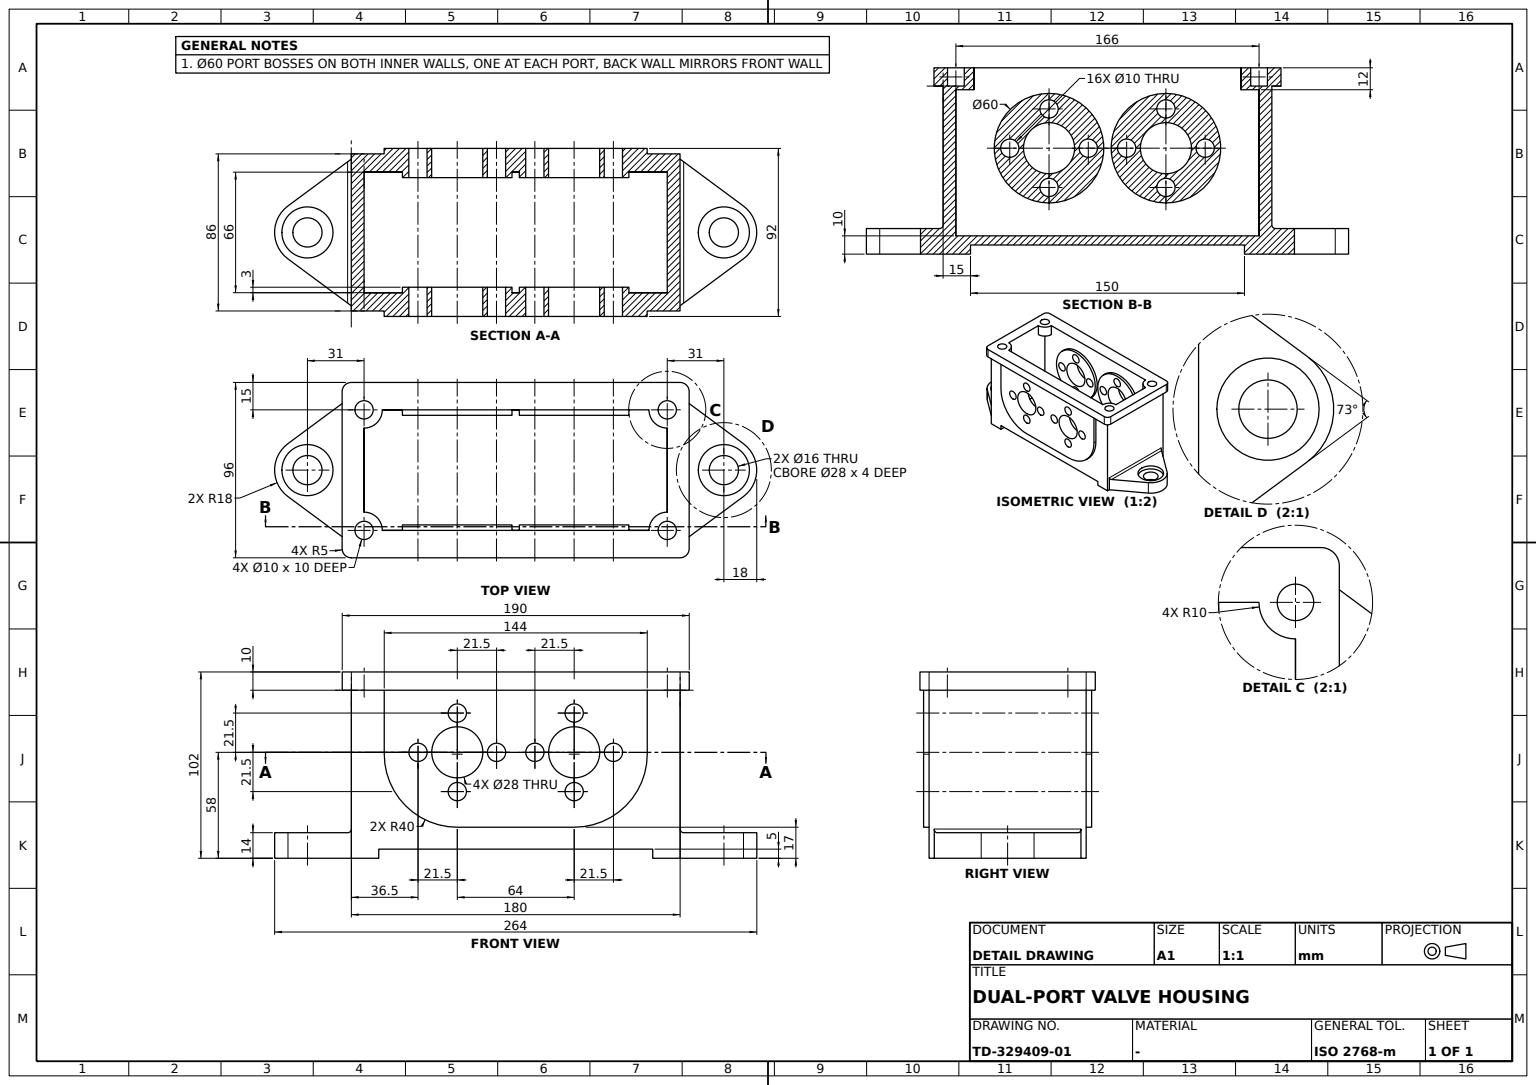
solid
v1 (-88,-33,92)
e1 v1 v1 CIRCLE(AX(P(-83,-33,92),D(0,0,-1),D(-1,0,0)),5) rev
face PLANE(AX(P(-83,-33,92),D(0,0,-1),D(-1,0,0))) rev [e1]
v2 (-90,-48,92)
v3 (-95,-43,92)
e2 v2 v3 CIRCLE(AX(P(-90,-43,92),D(0,0,1),D(1,0,0)),5) rev
v4 (-90,-48,102)
e3 v4 v2 LINE
v5 (-95,-43,102)
e4 v5 v4 CIRCLE(AX(P(-90,-43,102),D(0,0,1),D(1,0,0)),5)
e5 v3 v5 LINE
face CYL(AX(P(-90,-43,102),D(0,0,-1),D(-1,0,0)),5) [-e2 -e3 -e4 -e5]
v6 (-83,33,90)
v7 (-73,33,90)
e6 v6 v7 LINE
v8 (-83,23,90)
e7 v7 v8 CIRCLE(AX(P(-83,33,90),D(0,0,-1),D(1,0,0)),10)
e8 v8 v6 LINE
face PLANE(AX(P(-83,33,90),D(0,0,-1),D(-1,0,0))) [e6 e7 e8]
v9 (32,30,74.5)
e9 v9 v9 CIRCLE(AX(P(32,30,79.5),D(0,-1,0),D(0,0,-1)),5)
v10 (32,46,74.5)
e10 v10 v10 CIRCLE(AX(P(32,46,79.5),D(0,-1,0),D(0,0,-1)),5)
face CYL(AX(P(32,46,79.5),D(0,-1,0),D(0,0,-1)),5) rev [e9] [-e10]
v11 (100,0,14)
e11 v11 v11 CIRCLE(AX(P(114,0,14),D(0,0,-1),D(-1,0,0)),14)
v12 (100,0,10)
e12 v12 v12 CIRCLE(AX(P(114,0,10),D(0,0,-1),D(-1,0,0)),14) rev
face CYL(AX(P(114,0,14),D(0,0,-1),D(-1,0,0)),14) rev [-e11] [-e12]
v13 (53.5,30,53)
e13 v13 v13 CIRCLE(AX(P(53.5,30,58),D(0,-1,0),D(0,0,-1)),5)
v14 (53.5,46,53)
e14 v14 v14 CIRCLE(AX(P(53.5,46,58),D(0,-1,0),D(0,0,-1)),5)
face CYL(AX(P(53.5,46,58),D(0,-1,0),D(0,0,-1)),5) rev [e13] [-e14]
v15 (-95,43,102)
e15 v15 v5 LINE
v16 (-95,43,92)
e16 v15 v16 LINE
e17 v16 v3 LINE
face PLANE(AX(P(-95,48,102),D(1,0,0),D(0,0,-1))) rev [-e15 e16 e17 e5]
v17 (-32,30,31.5)
e18 v17 v17 CIRCLE(AX(P(-32,30,36.5),D(0,-1,0),D(0,0,-1)),5)
v18 (-32,30,74.5)
e19 v18 v18 CIRCLE(AX(P(-32,30,79.5),D(0,-1,0),D(0,0,-1)),5)
v19 (-10.5,30,53)
e20 v19 v19 CIRCLE(AX(P(-10.5,30,58),D(0,-1,0),D(0,0,-1)),5)
v20 (-32,30,72)
e21 v20 v20 CIRCLE(AX(P(-32,30,58),D(0,1,0),D(0,0,1)),14)
v21 (-53.5,30,53)
e22 v21 v21 CIRCLE(AX(P(-53.5,30,58),D(0,-1,0),D(0,0,-1)),5)
v22 (-2,30,58)
e23 v22 v22 CIRCLE(AX(P(-32,30,58),D(0,-1,0),D(1,0,0)),30)
face PLANE(AX(P(-32,30,58),D(0,-1,0),D(0,0,-1))) [-e18] [-e19] [-e20] [e21] [-e22] [e23]
v23 (73,33,90)
v24 (83,23,90)
e24 v23 v24 CIRCLE(AX(P(83,33,90),D(0,0,1),D(-1,0,0)),10)
v25 (83,23,102)
e25 v24 v25 LINE
v26 (73,33,102)
e26 v26 v25 CIRCLE(AX(P(83,33,102),D(0,0,1),D(-1,0,0)),10)
e27 v23 v26 LINE
face CYL(AX(P(83,33,90),D(0,0,1),D(1,0,0)),10) [e24 e25 -e26 -e27]
v27 (-122,0,10)
e28 v27 v27 CIRCLE(AX(P(-114,0,10),D(0,0,-1),D(-1,0,0)),8) rev
v28 (-128,0,10)
e29 v28 v28 CIRCLE(AX(P(-114,0,10),D(0,0,-1),D(-1,0,0)),14) rev
face PLANE(AX(P(-114,0,10),D(0,0,-1),D(-1,0,0))) rev [-e28] [e29]
v29 (78,-33,92)
e30 v29 v29 CIRCLE(AX(P(83,-33,92),D(0,0,-1),D(-1,0,0)),5) rev
face PLANE(AX(P(83,-33,92),D(0,0,-1),D(-1,0,0))) rev [e30]
v30 (-10.5,46,53)
e31 v30 v30 CIRCLE(AX(P(-10.5,46,58),D(0,-1,0),D(0,0,-1)),5)
face CYL(AX(P(-10.5,46,58),D(0,-1,0),D(0,0,-1)),5) rev [-e31] [e20]
v31 (-88,-33,102)
e32 v31 v31 CIRCLE(AX(P(-83,-33,102),D(0,0,-1),D(-1,0,0)),5)
face CYL(AX(P(-83,-33,102),D(0,0,-1),D(-1,0,0)),5) rev [-e32] [-e1]
v32 (90,-40.151112,0)
v33 (124.70681,-14.469423,0)
e33 v32 v33 LINE
v34 (124.70681,-14.469423,14)
e34 v34 v33 LINE
v35 (92,-38.67119,14)
e35 v35 v34 LINE
v36 (90,-40.151112,16)
e36 v35 v36 ELLIPSE(AX(P(92,-38.67119,16),D(-0.594822787,0.803856861,0),D(0.803856861,0.594822787,0)),2.488005,2)
e37 v36 v32 LINE
face PLANE(AX(P(90,-40.151112,14),D(-0.594822787,0.803856861,0),D(-0.803856861,-0.594822787,0))) rev [e33 -e34 -e35 e36 e37]
v37 (-73,-33,90)
v38 (-83,-23,90)
e38 v37 v38 CIRCLE(AX(P(-83,-33,90),D(0,0,1),D(1,0,0)),10)
v39 (-83,-33,90)
e39 v39 v37 LINE
e40 v38 v39 LINE
face PLANE(AX(P(-83,-33,90),D(0,0,1),D(1,0,0))) rev [-e38 -e39 -e40]
v40 (-90,48,92)
v41 (-90,48,102)
e41 v40 v41 LINE
v42 (90,48,102)
e42 v42 v41 LINE
v43 (90,48,92)
e43 v42 v43 LINE
e44 v43 v40 LINE
face PLANE(AX(P(95,48,102),D(0,-1,0),D(0,0,-1))) rev [e41 -e42 e43 e44]
v44 (83,33,90)
e45 v44 v23 LINE
e46 v24 v44 LINE
face PLANE(AX(P(83,33,90),D(0,0,1),D(1,0,0))) rev [-e24 -e45 -e46]
v45 (-124.70681,-14.469423,14)
v46 (-124.70681,14.469423,14)
e47 v45 v46 CIRCLE(AX(P(-114,0,14),D(0,0,-1),D(-1,0,0)),18)
v47 (-92,-38.67119,14)
e48 v47 v45 LINE
v48 (-92,38.67119,14)
e49 v47 v48 LINE
e50 v46 v48 LINE
v49 (-128,0,14)
e51 v49 v49 CIRCLE(AX(P(-114,0,14),D(0,0,-1),D(-1,0,0)),14)
face PLANE(AX(P(-114,0,14),D(0,0,-1),D(-1,0,0))) rev [-e47 -e48 e49 -e50] [e51]
v50 (-32,-46,17)
v51 (-32,-43,17)
e52 v50 v51 LINE
v52 (-72,-46,57)
e53 v52 v50 CIRCLE(AX(P(-32,-46,57),D(0,-1,0),D(1,0,0)),40)
v53 (-72,-43,57)
e54 v52 v53 LINE
e55 v51 v53 CIRCLE(AX(P(-32,-43,57),D(0,-1,0),D(0,0,-1)),40) rev
face CYL(AX(P(-32,-46,57),D(0,1,0),D(0,0,1)),40) [-e52 -e53 e54 -e55]
v54 (90,-48,102)
v55 (95,-43,102)
e56 v54 v55 CIRCLE(AX(P(90,-43,102),D(0,0,1),D(1,0,0)),5)
v56 (90,-48,92)
e57 v56 v54 LINE
v57 (95,-43,92)
e58 v57 v56 CIRCLE(AX(P(90,-43,92),D(0,0,1),D(1,0,0)),5) rev
e59 v55 v57 LINE
face CYL(AX(P(90,-43,102),D(0,0,-1),D(-1,0,0)),5) [-e56 -e57 -e58 -e59]
v58 (124.70681,14.469423,0)
v59 (90,40.151112,0)
e60 v58 v59 LINE
v60 (90,40.151112,16)
e61 v60 v59 LINE
v61 (92,38.67119,14)
e62 v60 v61 ELLIPSE(AX(P(92,38.67119,16),D(-0.594822787,-0.803856861,0),D(-0.803856861,0.594822787,0)),2.488005,2)
v62 (124.70681,14.469423,14)
e63 v62 v61 LINE
e64 v62 v58 LINE
face PLANE(AX(P(124.70681,14.469423,14),D(-0.594822787,-0.803856861,0),D(0.803856861,-0.594822787,0))) rev [e60 -e61 e62 -e63 e64]
v63 (-73,-33,102)
e65 v37 v63 LINE
v64 (-83,-23,102)
e66 v38 v64 LINE
e67 v63 v64 CIRCLE(AX(P(-83,-33,102),D(0,0,1),D(1,0,0)),10)
face CYL(AX(P(-83,-33,90),D(0,0,1),D(1,0,0)),10) [-e65 e38 e66 -e67]
v65 (-32,-30,74.5)
e68 v65 v65 CIRCLE(AX(P(-32,-30,79.5),D(0,-1,0),D(0,0,-1)),5)
v66 (-32,-46,74.5)
e69 v66 v66 CIRCLE(AX(P(-32,-46,79.5),D(0,-1,0),D(0,0,-1)),5)
face CYL(AX(P(-32,46,79.5),D(0,-1,0),D(0,0,-1)),5) rev [-e68] [e69]
v67 (-32,-33,28)
e70 v67 v67 CIRCLE(AX(P(-32,-33,58),D(0,-1,0),D(0,0,-1)),30)
v68 (32,-33,28)
e71 v68 v68 CIRCLE(AX(P(32,-33,58),D(0,-1,0),D(0,0,-1)),30)
v69 (83,-33,10)
v70 (83,-33,90)
e72 v69 v70 LINE
v71 (-83,-33,10)
e73 v71 v69 LINE
e74 v71 v39 LINE
v72 (73,-33,102)
e75 v63 v72 LINE
v73 (73,-33,90)
e76 v73 v72 LINE
e77 v70 v73 LINE
face PLANE(AX(P(83,-33,123),D(0,-1,0),D(0,0,-1))) rev [e70] [e71] [-e72 -e73 e74 e39 e65 e75 -e76 -e77]
v74 (32,-30,74.5)
e78 v74 v74 CIRCLE(AX(P(32,-30,79.5),D(0,-1,0),D(0,0,-1)),5)
v75 (32,-46,74.5)
e79 v75 v75 CIRCLE(AX(P(32,-46,79.5),D(0,-1,0),D(0,0,-1)),5)
face CYL(AX(P(32,46,79.5),D(0,-1,0),D(0,0,-1)),5) rev [-e78] [e79]
v76 (62,-30,58)
e80 v76 v76 CIRCLE(AX(P(32,-30,58),D(0,-1,0),D(1,0,0)),30)
face CYL(AX(P(32,-30,58),D(0,-1,0),D(0,0,-1)),30) [e80] [-e71]
v77 (-88,33,92)
e81 v77 v77 CIRCLE(AX(P(-83,33,92),D(0,0,-1),D(-1,0,0)),5) rev
face PLANE(AX(P(-83,33,92),D(0,0,-1),D(-1,0,0))) rev [e81]
v78 (-72,-46,92)
e82 v78 v52 LINE
v79 (-72,-43,92)
e83 v78 v79 LINE
e84 v53 v79 LINE
face PLANE(AX(P(-72,-46,92),D(1,0,0),D(0,0,-1))) rev [-e82 e83 -e84 -e54]
v80 (95,43,92)
e85 v57 v80 LINE
v81 (95,43,102)
e86 v80 v81 LINE
e87 v55 v81 LINE
face PLANE(AX(P(95,-48,102),D(-1,0,0),D(0,0,1))) rev [e85 e86 -e87 e59]
v82 (106,0,10)
e88 v82 v82 CIRCLE(AX(P(114,0,10),D(0,0,-1),D(-1,0,0)),8) rev
face PLANE(AX(P(114,0,10),D(0,0,-1),D(-1,0,0))) rev [-e88] [e12]
v83 (106,0,0)
e89 v83 v83 CIRCLE(AX(P(114,0,0),D(0,0,-1),D(-1,0,0)),8)
face CYL(AX(P(114,0,-67.414906),D(0,0,-1),D(-1,0,0)),8) rev [e89] [e88]
v84 (-2,-30,58)
e90 v84 v84 CIRCLE(AX(P(-32,-30,58),D(0,-1,0),D(1,0,0)),30)
v85 (-10.5,-30,53)
e91 v85 v85 CIRCLE(AX(P(-10.5,-30,58),D(0,-1,0),D(0,0,-1)),5)
v86 (-53.5,-30,53)
e92 v86 v86 CIRCLE(AX(P(-53.5,-30,58),D(0,-1,0),D(0,0,-1)),5)
v87 (-32,-30,44)
e93 v87 v87 CIRCLE(AX(P(-32,-30,58),D(0,-1,0),D(0,0,-1)),14)
v88 (-32,-30,31.5)
e94 v88 v88 CIRCLE(AX(P(-32,-30,36.5),D(0,-1,0),D(0,0,-1)),5)
face PLANE(AX(P(-32,-30,58),D(0,-1,0),D(0,0,-1))) rev [-e90] [e91] [e92] [e93] [e68] [e94]
v89 (-90,40.151112,0)
v90 (-90,43,0)
e95 v89 v90 LINE
v91 (-75,43,0)
e96 v90 v91 LINE
v92 (-75,-43,0)
e97 v92 v91 LINE
v93 (-90,-43,0)
e98 v92 v93 LINE
v94 (-90,-40.151112,0)
e99 v93 v94 LINE
v95 (-124.70681,-14.469423,0)
e100 v94 v95 LINE
v96 (-124.70681,14.469423,0)
e101 v95 v96 CIRCLE(AX(P(-114,0,0),D(0,0,-1),D(-1,0,0)),18)
e102 v96 v89 LINE
v97 (-122,0,0)
e103 v97 v97 CIRCLE(AX(P(-114,0,0),D(0,0,-1),D(-1,0,0)),8)
face PLANE(AX(P(0,0,0),D(0,0,-1),D(-1,0,0))) [e95 e96 -e97 e98 e99 e100 e101 e102] [-e103]
e104 v33 v58 CIRCLE(AX(P(114,0,0),D(0,0,1),D(1,0,0)),18)
v98 (90,-43,0)
e105 v32 v98 LINE
v99 (75,-43,0)
e106 v98 v99 LINE
v100 (75,43,0)
e107 v100 v99 LINE
v101 (90,43,0)
e108 v100 v101 LINE
e109 v101 v59 LINE
face PLANE(AX(P(0,0,0),D(0,0,-1),D(-1,0,0))) [-e89] [-e104 -e33 e105 e106 -e107 e108 e109 -e60]
v102 (32,46,44)
e110 v102 v102 CIRCLE(AX(P(32,46,58),D(0,-1,0),D(0,0,-1)),14)
v103 (32,30,72)
e111 v103 v103 CIRCLE(AX(P(32,30,58),D(0,1,0),D(0,0,1)),14)
face CYL(AX(P(32,30,58),D(0,1,0),D(0,0,1)),14) rev [-e110] [-e111]
e112 v2 v56 LINE
e113 v4 v54 LINE
face PLANE(AX(P(-95,-48,102),D(0,1,0),D(0,0,1))) rev [e112 e57 -e113 e3]
v104 (-32,46,74.5)
e114 v104 v104 CIRCLE(AX(P(-32,46,79.5),D(0,-1,0),D(0,0,-1)),5)
face CYL(AX(P(-32,46,79.5),D(0,-1,0),D(0,0,-1)),5) rev [e19] [-e114]
v105 (83,-23,90)
e115 v73 v105 CIRCLE(AX(P(83,-33,90),D(0,0,-1),D(-1,0,0)),10)
e116 v105 v70 LINE
face PLANE(AX(P(83,-33,90),D(0,0,-1),D(-1,0,0))) [e77 e115 e116]
face CYL(AX(P(-114,0,-67.414906),D(0,0,-1),D(-1,0,0)),8) rev [e28] [e103]
v106 (-32,-46,31.5)
e117 v106 v106 CIRCLE(AX(P(-32,-46,36.5),D(0,-1,0),D(0,0,-1)),5)
face CYL(AX(P(-32,46,36.5),D(0,-1,0),D(0,0,-1)),5) rev [-e94] [e117]
v107 (-72,46,57)
v108 (-32,46,17)
e118 v107 v108 CIRCLE(AX(P(-32,46,57),D(0,-1,0),D(1,0,0)),40)
v109 (-32,43,17)
e119 v109 v108 LINE
v110 (-72,43,57)
e120 v110 v109 CIRCLE(AX(P(-32,43,57),D(0,1,0),D(0,0,1)),40) rev
e121 v110 v107 LINE
face CYL(AX(P(-32,-46,57),D(0,1,0),D(0,0,1)),40) [e118 -e119 -e120 e121]
v111 (-88,33,102)
e122 v111 v111 CIRCLE(AX(P(-83,33,102),D(0,0,-1),D(-1,0,0)),5)
v112 (-73,33,102)
e123 v26 v112 LINE
v113 (83,-23,102)
e124 v113 v25 LINE
e125 v72 v113 CIRCLE(AX(P(83,-33,102),D(0,0,-1),D(-1,0,0)),10)
v114 (-83,23,102)
e126 v114 v64 LINE
e127 v112 v114 CIRCLE(AX(P(-83,33,102),D(0,0,-1),D(1,0,0)),10)
v115 (78,-33,102)
e128 v115 v115 CIRCLE(AX(P(83,-33,102),D(0,0,-1),D(-1,0,0)),5)
v116 (78,33,102)
e129 v116 v116 CIRCLE(AX(P(83,33,102),D(0,0,-1),D(-1,0,0)),5)
e130 v81 v42 CIRCLE(AX(P(90,43,102),D(0,0,1),D(1,0,0)),5)
e131 v41 v15 CIRCLE(AX(P(-90,43,102),D(0,0,1),D(1,0,0)),5)
face PLANE(AX(P(0,0,102),D(0,0,1),D(1,0,0))) [e32] [e122] [-e123 e26 -e124 -e125 -e75 e67 -e126 -e127] [e128] [e129] [e130 e42 e131 e15 e4 e113 e56 e87]
e132 v16 v40 CIRCLE(AX(P(-90,43,92),D(0,0,1),D(1,0,0)),5) rev
e133 v43 v80 CIRCLE(AX(P(90,43,92),D(0,0,1),D(1,0,0)),5) rev
v117 (-90,43,92)
v118 (-72,43,92)
e134 v117 v118 LINE
v119 (-90,-43,92)
e135 v119 v117 LINE
e136 v79 v119 LINE
v120 (72,-46,92)
e137 v120 v78 LINE
v121 (72,-43,92)
e138 v120 v121 LINE
v122 (90,-43,92)
e139 v122 v121 LINE
v123 (90,43,92)
e140 v123 v122 LINE
v124 (72,43,92)
e141 v124 v123 LINE
v125 (72,46,92)
e142 v124 v125 LINE
v126 (-72,46,92)
e143 v125 v126 LINE
e144 v118 v126 LINE
face PLANE(AX(P(0,0,92),D(0,0,1),D(1,0,0))) rev [-e112 e2 -e17 e132 -e44 e133 -e85 e58] [-e134 -e135 -e136 -e83 -e137 e138 -e139 -e140 -e141 e142 e143 -e144]
e145 v123 v101 LINE
v127 (75,43,5)
e146 v127 v100 LINE
v128 (-75,43,5)
e147 v128 v127 LINE
e148 v91 v128 LINE
e149 v117 v90 LINE
e150 v118 v110 LINE
v129 (32,43,17)
e151 v109 v129 LINE
v130 (72,43,57)
e152 v129 v130 CIRCLE(AX(P(32,43,57),D(0,1,0),D(0,0,1)),40) rev
e153 v130 v124 LINE
face PLANE(AX(P(-90,43,92),D(0,1,0),D(0,0,1))) [e145 -e108 -e146 -e147 -e148 -e96 -e149 e134 e150 e120 e151 e152 e153 e141]
v131 (32,46,17)
e154 v129 v131 LINE
v132 (72,46,57)
e155 v131 v132 CIRCLE(AX(P(32,46,57),D(0,-1,0),D(1,0,0)),40)
e156 v130 v132 LINE
face CYL(AX(P(32,-46,57),D(0,1,0),D(0,0,1)),40) [e154 e155 -e156 -e152]
e157 v34 v62 CIRCLE(AX(P(114,0,14),D(0,0,1),D(1,0,0)),18)
e158 v61 v35 LINE
face PLANE(AX(P(114,0,14),D(0,0,1),D(1,0,0))) [e11] [e157 e63 e158 e35]
v133 (10.5,46,53)
e159 v133 v133 CIRCLE(AX(P(10.5,46,58),D(0,-1,0),D(0,0,-1)),5)
v134 (10.5,30,53)
e160 v134 v134 CIRCLE(AX(P(10.5,30,58),D(0,-1,0),D(0,0,-1)),5)
face CYL(AX(P(10.5,46,58),D(0,-1,0),D(0,0,-1)),5) rev [-e159] [e160]
face CYL(AX(P(-32,-30,58),D(0,-1,0),D(0,0,-1)),30) [e90] [-e70]
v135 (78,33,92)
e161 v135 v135 CIRCLE(AX(P(83,33,92),D(0,0,-1),D(-1,0,0)),5) rev
face CYL(AX(P(83,33,102),D(0,0,-1),D(-1,0,0)),5) rev [-e129] [-e161]
e162 v8 v114 LINE
e163 v7 v112 LINE
face CYL(AX(P(-83,33,90),D(0,0,1),D(1,0,0)),10) [e127 -e162 -e7 e163]
v136 (-75,-43,5)
e164 v128 v136 LINE
v137 (75,-43,5)
e165 v127 v137 LINE
e166 v137 v136 LINE
face PLANE(AX(P(-75,-50,5),D(0,0,1),D(1,0,0))) rev [-e164 e147 e165 e166]
v138 (72,-46,57)
e167 v138 v120 LINE
v139 (72,-43,57)
e168 v138 v139 LINE
e169 v121 v139 LINE
face PLANE(AX(P(72,-46,57),D(-1,0,0),D(0,0,1))) rev [-e138 -e167 e168 -e169]
v140 (32,-46,17)
e170 v50 v140 LINE
v141 (32,-43,17)
e171 v141 v51 LINE
e172 v140 v141 LINE
face PLANE(AX(P(-32,-46,17),D(0,0,1),D(1,0,0))) rev [-e170 e52 -e171 -e172]
e173 v126 v107 LINE
face PLANE(AX(P(-72,-46,92),D(1,0,0),D(0,0,-1))) rev [e173 -e121 -e150 e144]
e174 v108 v131 LINE
face PLANE(AX(P(-32,-46,17),D(0,0,1),D(1,0,0))) rev [-e154 -e151 e119 e174]
v142 (-53.5,46,53)
e175 v142 v142 CIRCLE(AX(P(-53.5,46,58),D(0,-1,0),D(0,0,-1)),5)
v143 (-32,46,44)
e176 v143 v143 CIRCLE(AX(P(-32,46,58),D(0,-1,0),D(0,0,-1)),14)
v144 (-32,46,31.5)
e177 v144 v144 CIRCLE(AX(P(-32,46,36.5),D(0,-1,0),D(0,0,-1)),5)
v145 (32,46,31.5)
e178 v145 v145 CIRCLE(AX(P(32,46,36.5),D(0,-1,0),D(0,0,-1)),5)
e179 v132 v125 LINE
face PLANE(AX(P(-32,46,57),D(0,-1,0),D(0,0,-1))) rev [e10] [e31] [e175] [e176] [e177] [e14] [e159] [e110] [e178] [-e174 -e118 -e173 -e143 -e179 -e155] [e114]
face CYL(AX(P(-53.5,46,58),D(0,-1,0),D(0,0,-1)),5) rev [e22] [-e175]
e180 v36 v60 LINE
e181 v122 v98 LINE
face PLANE(AX(P(90,43,92),D(1,0,0),D(0,0,-1))) [-e37 e180 e61 -e109 -e145 e140 e181 -e105]
v146 (-32,33,88)
e182 v146 v146 CIRCLE(AX(P(-32,33,58),D(0,1,0),D(0,0,1)),30)
face CYL(AX(P(-32,43,58),D(0,-1,0),D(0,0,-1)),30) [-e23] [-e182]
v147 (10.5,-46,53)
e183 v147 v147 CIRCLE(AX(P(10.5,-46,58),D(0,-1,0),D(0,0,-1)),5)
v148 (10.5,-30,53)
e184 v148 v148 CIRCLE(AX(P(10.5,-30,58),D(0,-1,0),D(0,0,-1)),5)
face CYL(AX(P(10.5,46,58),D(0,-1,0),D(0,0,-1)),5) rev [e183] [-e184]
face CYL(AX(P(-32,30,58),D(0,1,0),D(0,0,1)),14) rev [-e176] [-e21]
face CYL(AX(P(-90,43,102),D(0,0,-1),D(-1,0,0)),5) [-e131 -e41 -e132 -e16]
face CYL(AX(P(83,-33,102),D(0,0,-1),D(-1,0,0)),5) rev [-e128] [-e30]
v149 (-53.5,-46,53)
e185 v149 v149 CIRCLE(AX(P(-53.5,-46,58),D(0,-1,0),D(0,0,-1)),5)
face CYL(AX(P(-53.5,46,58),D(0,-1,0),D(0,0,-1)),5) rev [-e92] [e185]
v150 (-10.5,-46,53)
e186 v150 v150 CIRCLE(AX(P(-10.5,-46,58),D(0,-1,0),D(0,0,-1)),5)
face CYL(AX(P(-10.5,46,58),D(0,-1,0),D(0,0,-1)),5) rev [e186] [-e91]
e187 v99 v137 LINE
e188 v139 v141 CIRCLE(AX(P(32,-43,57),D(0,-1,0),D(0,0,-1)),40) rev
e189 v119 v93 LINE
e190 v136 v92 LINE
face PLANE(AX(P(90,-43,92),D(0,-1,0),D(0,0,-1))) [-e166 -e187 -e106 -e181 e139 e169 e188 e171 e55 e84 e136 e189 -e98 -e190]
v151 (-83,33,10)
e191 v151 v6 LINE
v152 (83,33,10)
e192 v152 v151 LINE
e193 v152 v44 LINE
v153 (32,33,88)
e194 v153 v153 CIRCLE(AX(P(32,33,58),D(0,1,0),D(0,0,1)),30)
face PLANE(AX(P(-83,33,123),D(0,1,0),D(0,0,1))) rev [e45 e27 e123 -e163 -e6 -e191 -e192 e193] [e182] [e194]
e195 v140 v138 CIRCLE(AX(P(32,-46,57),D(0,-1,0),D(1,0,0)),40)
face CYL(AX(P(32,-46,57),D(0,1,0),D(0,0,1)),40) [-e168 -e195 e172 -e188]
v154 (-90,40.151112,16)
e196 v154 v89 LINE
v155 (-90,-40.151112,16)
e197 v154 v155 LINE
e198 v155 v94 LINE
face PLANE(AX(P(-90,-43,92),D(-1,0,0),D(0,0,1))) [-e95 -e196 e197 e198 -e99 -e189 e135 e149]
face CYL(AX(P(114,0,14),D(0,0,-1),D(-1,0,0)),18) [-e157 e34 e104 -e64]
v156 (32,-46,31.5)
e199 v156 v156 CIRCLE(AX(P(32,-46,36.5),D(0,-1,0),D(0,0,-1)),5)
v157 (32,-46,44)
e200 v157 v157 CIRCLE(AX(P(32,-46,58),D(0,-1,0),D(0,0,-1)),14)
v158 (53.5,-46,53)
e201 v158 v158 CIRCLE(AX(P(53.5,-46,58),D(0,-1,0),D(0,0,-1)),5)
v159 (-32,-46,44)
e202 v159 v159 CIRCLE(AX(P(-32,-46,58),D(0,-1,0),D(0,0,-1)),14)
face PLANE(AX(P(-32,-46,57),D(0,-1,0),D(0,0,-1))) [-e183] [-e79] [-e117] [-e185] [-e186] [e195 e167 e137 e82 e53 e170] [-e199] [-e200] [-e201] [-e202] [-e69]
v160 (32,30,31.5)
e203 v160 v160 CIRCLE(AX(P(32,30,36.5),D(0,-1,0),D(0,0,-1)),5)
v161 (62,30,58)
e204 v161 v161 CIRCLE(AX(P(32,30,58),D(0,-1,0),D(1,0,0)),30)
face PLANE(AX(P(32,30,58),D(0,-1,0),D(0,0,-1))) [-e13] [-e160] [-e203] [-e9] [e111] [e204]
v162 (32,-30,44)
e205 v162 v162 CIRCLE(AX(P(32,-30,58),D(0,-1,0),D(0,0,-1)),14)
face CYL(AX(P(32,-30,58),D(0,-1,0),D(0,0,-1)),14) rev [e200] [-e205]
v163 (32,-30,31.5)
e206 v163 v163 CIRCLE(AX(P(32,-30,36.5),D(0,-1,0),D(0,0,-1)),5)
face CYL(AX(P(32,46,36.5),D(0,-1,0),D(0,0,-1)),5) rev [-e206] [e199]
face CYL(AX(P(32,46,36.5),D(0,-1,0),D(0,0,-1)),5) rev [-e178] [e203]
face PLANE(AX(P(-75,-50,-10),D(-1,0,0),D(0,0,1))) rev [e97 e148 e164 e190]
e207 v48 v154 ELLIPSE(AX(P(-92,38.67119,16),D(-0.594822787,0.803856861,0),D(-0.803856861,-0.594822787,0)),2.488005,2) rev
e208 v46 v96 LINE
face PLANE(AX(P(-124.70681,14.469423,14),D(-0.594822787,0.803856861,0),D(-0.803856861,-0.594822787,0))) [e50 e207 e196 -e102 -e208]
e209 v105 v113 LINE
face CYL(AX(P(83,-33,90),D(0,0,1),D(1,0,0)),10) [e76 e125 -e209 -e115]
face CYL(AX(P(-32,46,36.5),D(0,-1,0),D(0,0,-1)),5) rev [-e177] [e18]
e210 v45 v95 LINE
face CYL(AX(P(-114,0,14),D(0,0,-1),D(-1,0,0)),18) [-e210 e47 e208 -e101]
face CYL(AX(P(92,0,16),D(0,1,0),D(0,0,1)),2) rev [-e180 -e36 -e158 -e62]
face CYL(AX(P(-32,-30,58),D(0,-1,0),D(0,0,-1)),14) rev [e202] [-e93]
face PLANE(AX(P(83,33,92),D(0,0,-1),D(-1,0,0))) rev [e161]
e211 v69 v152 LINE
e212 v151 v71 LINE
face PLANE(AX(P(0,0,10),D(0,0,-1),D(-1,0,0))) rev [e211 e192 e212 e73]
e213 v155 v47 ELLIPSE(AX(P(-92,-38.67119,16),D(-0.594822787,-0.803856861,0),D(0.803856861,-0.594822787,0)),2.488005,2) rev
face CYL(AX(P(-92,-43,16),D(0,-1,0),D(0,0,-1)),2) rev [-e213 -e197 -e207 -e49]
face CYL(AX(P(-83,33,102),D(0,0,-1),D(-1,0,0)),5) rev [-e122] [-e81]
face PLANE(AX(P(-83,-33,123),D(-1,0,0),D(0,0,1))) rev [e126 -e66 e40 -e74 -e212 e191 -e8 e162]
face PLANE(AX(P(72,-46,57),D(-1,0,0),D(0,0,1))) rev [e156 e179 -e142 -e153]
face PLANE(AX(P(-90,-40.151112,14),D(-0.594822787,-0.803856861,0),D(0.803856861,-0.594822787,0))) [-e100 -e198 e213 e48 e210]
v164 (53.5,-30,53)
e214 v164 v164 CIRCLE(AX(P(53.5,-30,58),D(0,-1,0),D(0,0,-1)),5)
face CYL(AX(P(53.5,46,58),D(0,-1,0),D(0,0,-1)),5) rev [-e214] [e201]
face CYL(AX(P(32,43,58),D(0,-1,0),D(0,0,-1)),30) [-e204] [-e194]
face PLANE(AX(P(75,-50,5),D(1,0,0),D(0,0,-1))) rev [e107 e187 -e165 e146]
face PLANE(AX(P(83,33,123),D(1,0,0),D(0,0,-1))) rev [-e193 -e211 e72 -e116 e209 e124 -e25 e46]
face CYL(AX(P(-114,0,14),D(0,0,-1),D(-1,0,0)),14) rev [-e51] [-e29]
face PLANE(AX(P(32,-30,58),D(0,-1,0),D(0,0,-1))) rev [e206] [e184] [e205] [-e80] [e78] [e214]
face CYL(AX(P(90,43,102),D(0,0,-1),D(-1,0,0)),5) [-e130 -e86 -e133 -e43]
